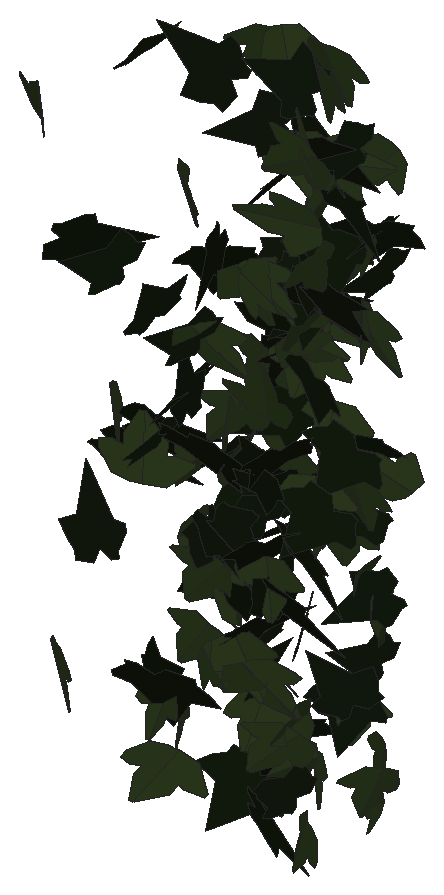
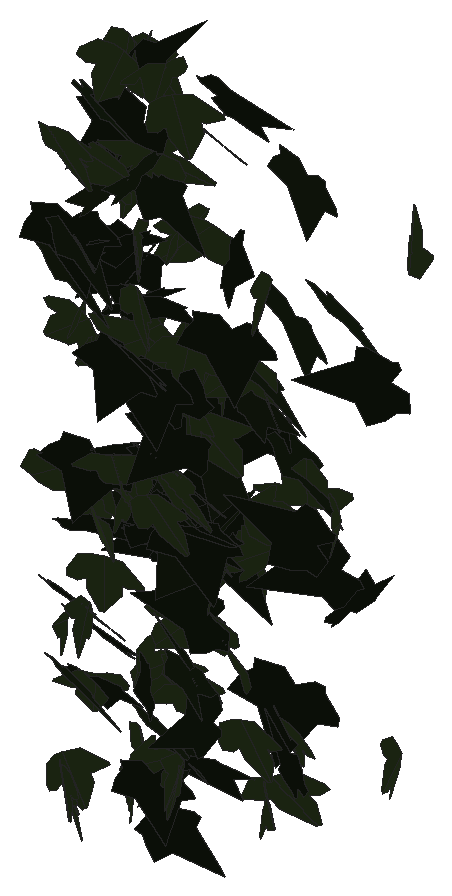
# SketchUp Ruby script. Lengths in inches.
U = 1.inch
M = Sketchup.active_model
def pt(a) = Geom::Point3d.new(a.map { |v| v * U })
def face(e, loops, mat)
  f = e.add_face(loops[0].map { |a| pt(a) })
  loops[1..].each { |l| e.add_face(l.map { |a| pt(a) }).erase! }
  f.material = f.back_material = mat if mat
  f
end
# faces: each face lists its corners as indices into pts; further lists are holes
def faces(e, pts, list, mat = nil) = list.each { |f| face(e, (f[0].is_a?(Array) ? f : [f]).map { |l| l.map { |i| pts[i] } }, mat) }
# xy, xz, yz: faces in a plane at the given z, y or x. An outline is a flat list of corners, or four numbers for a rectangle; further outlines are holes
def ring(l) = l.size == 4 ? [[l[0], l[1]], [l[2], l[1]], [l[2], l[3]], [l[0], l[3]]] : l.each_slice(2).to_a
def flat(e, list, mat, &to3) = list.each { |f| face(e, (f[0].is_a?(Array) ? f : [f]).map { |l| ring(l).map { |u, v| to3.(u, v) } }, mat) }
def xy(e, z, list, mat = nil) = flat(e, list, mat) { |x, y| [x, y, z] }
def xz(e, y, list, mat = nil) = flat(e, list, mat) { |x, z| [x, y, z] }
def yz(e, x, list, mat = nil) = flat(e, list, mat) { |y, z| [x, y, z] }
def lines(e, pts, list) = list.each { |a, b| e.add_line(pt(pts[a]), pt(pts[b])) }
# prism: a flat outline (further loops are holes) pulled along v
def prism(e, loops, v, mat = nil)
  f = face(e, loops, mat); d = Geom::Vector3d.new(v.map { |x| x * U })
  f.pushpull(f.normal.samedirection?(d) ? d.length : -d.length)
end
def box(e, o, s, mat = nil) = prism(e, [[o, [o[0] + s[0], o[1], o[2]], [o[0] + s[0], o[1] + s[1], o[2]], [o[0], o[1] + s[1], o[2]]]], [0, 0, s[2]], mat)
def at(x, y, z, deg = 0) = Geom::Transformation.translation(pt([x, y, z])) * Geom::Transformation.rotation(ORIGIN, Z_AXIS, deg.degrees)
def axes(o, x, y, z) = Geom::Transformation.new([*x, 0, *y, 0, *z, 0, *pt(o).to_a, 1])
def part(name) = M.definitions.add(name)
# library, detail: a bought-in or finely detailed component or shape, given as its bounding box
def library(name, o, s) = part(name).tap { |d| box(d.entities, o, s) }
def detail(e, o, s) = box(e.add_group.entities, o, s)
def put(e, d, t, mat = nil) = e.add_instance(d, t).tap { |i| i.material = mat if mat }
def group(e, t, mat = nil) = e.add_group.tap { |g| g.transformation = t; g.material = mat if mat }.entities
root = M.entities
M.materials.add("1026 AP 7946 SUNNY SIDE UP").color = [254, 231, 186]
M.materials.add("efeu1").color = [18, 25, 13]
M.materials.add("efeu2").color = [43, 57, 29]
c1 = part("ivyleaf_9")
p = [[1.54,2.16,1.25],[1.36,2.04,1.19],[-0.21,0.99,0.68],[-0.71,1.11,0.82],[-0.85,0.86,0.67],[-0.8,0.17,0.21],
  [-0.9,-0.01,0.1],[-0.67,-0.16,-0.02],[-0.08,-0.08,-0.05],[-0.03,-0.6,-0.4],[0.65,-0.88,-0.66],[0.83,-0.6,-0.49],
  [1.29,-0.42,-0.43],[1.8125,-0.07,-0.26],[1.21,0.44,0.15]]
faces(c1.entities,p,[[0,1,2,3,4,5,6,7,8,9,10,11,12,13,14]],"efeu1")
c2 = part("ivyleaf_10")
p = [[0,0.5,-0.03],[-0.0625,2.02,-0.43],[-0.19,2.01,-0.46],[-0.54,1.05,-0.29],[-0.52,0.625,-0.18],[-0.83,0.76,-0.28],
  [-1.16,0.64,-0.33],[-1.15,0.33,-0.24],[-0.77,-0.39,0.02],[-0.3,-0.51,0.16],[0.04,-0.48,0.23],[-0.02,2.01,-0.4375],
  [-0.06,2.01,-0.43],[0.04,-0.49,0.23],[0.67,-0.49,0.14],[1.38,0.36,-0.2],[1.375,0.51,-0.24],[0.81,0.65,-0.19],
  [0.62,0.59,-0.15],[0.6,1.09,-0.28],[0.5,1.23,-0.31]]
faces(c2.entities,p,[[0,1,2,3,4,5,6,7,8,9,10],[11,12,0,13,14,15,16,17,18,19,20]],"efeu2")
put(root,c1,axes([97.57,211.43,285.4],[-0.02383,0.29282,-0.12965],[0.02278,-0.12438,-0.3155],[-0.53994,-0.01817,-0.00759]),"1026 AP 7946 SUNNY SIDE UP")
put(root,c1,axes([96.1,211.34,285.11],[0.5804,0.06021,-0.09484],[-0.15726,0.01233,-0.37035],[-0.09346,0.35318,0.03417]),"1026 AP 7946 SUNNY SIDE UP")
put(root,c1,axes([95.49,211.43,284.89],[-0.25342,0.29453,-0.03914],[0.00462,-0.04385,-0.35364],[-0.50464,-0.14831,0.01642]),"1026 AP 7946 SUNNY SIDE UP")
put(root,c1,axes([95.49,211.38,281.24],[0.47591,0.14978,-0.1513],[-0.20633,-0.07643,-0.34121],[-0.28502,0.30543,-0.00564]),"1026 AP 7946 SUNNY SIDE UP")
put(root,c2,axes([97.57,211.62,280.87],[-0.33154,-0.14288,0.2048],[-0.19603,-0.16247,-0.25593],[0.35766,-0.2215,0.04957]),"1026 AP 7946 SUNNY SIDE UP")
put(root,c1,axes([94.84,211.4,287.32],[-0.2851,0.26757,0.10404],[-0.1298,0.06211,-0.33577],[-0.46342,-0.18201,0.03004]),"1026 AP 7946 SUNNY SIDE UP")
put(root,c2,axes([96.43,211.53,283.13],[-0.47339,-0.03717,0.17911],[-0.26834,-0.07,-0.29885],[0.11445,-0.31784,0.04016]),"1026 AP 7946 SUNNY SIDE UP")
put(root,c2,axes([95.54,211.59,279.86],[0.45236,0.12368,-0.16682],[-0.23003,-0.08151,-0.31525],[-0.25018,0.29859,-0.01177]),"1026 AP 7946 SUNNY SIDE UP")
put(root,c2,axes([97.2,211.57,283.4],[0.50584,-0.01989,0.0995],[0.15538,-0.0254,-0.31947],[0.04502,0.31118,-0.01533]),"1026 AP 7946 SUNNY SIDE UP")
put(root,c2,axes([93.66,211.55,280.87],[-0.26233,0.27662,-0.11767],[0.04788,-0.11372,-0.33938],[-0.50531,-0.15438,0.02893]),"1026 AP 7946 SUNNY SIDE UP")
put(root,c2,axes([97.07,211.49,281.8],[-0.42943,-0.09787,-0.19649],[0.31475,0.02044,-0.28698],[0.15577,-0.31112,0.03817]),"1026 AP 7946 SUNNY SIDE UP")
put(root,c1,axes([97.17,211.46,279.73],[0.39889,-0.1767,-0.18172],[-0.20291,0.11898,-0.31235],[0.35999,0.26286,0.02531]),"1026 AP 7946 SUNNY SIDE UP")
put(root,c2,axes([97.97,211.51,290.03],[-0.35651,0.0191,0.27204],[-0.43213,-0.01927,-0.22418],[0.00462,-0.32891,0.02431]),"1026 AP 7946 SUNNY SIDE UP")
put(root,c2,axes([97.98,211.51,279.65],[-0.29823,0.25671,0.06959],[-0.22701,-0.02267,-0.3072],[-0.38643,-0.1848,0.12676]),"1026 AP 7946 SUNNY SIDE UP")
put(root,c1,axes([97.26,211.47,284.99],[0.0507,-0.00402,-0.33283],[-0.52764,-0.00502,-0.03198],[-0.00784,0.31222,-0.00044]),"1026 AP 7946 SUNNY SIDE UP")
put(root,c2,axes([96.73,211.35,285.44],[0.14773,-0.03586,0.33108],[-0.3063,0.25646,0.08964],[-0.43165,-0.19425,0.0497]),"1026 AP 7946 SUNNY SIDE UP")
put(root,c2,axes([95.38,211.64,280.81],[0.39832,-0.18079,0.05152],[0.04098,-0.05103,-0.31979],[0.29252,0.25332,-0.02535]),"1026 AP 7946 SUNNY SIDE UP")
put(root,c1,axes([97.26,211.49,283.84],[0.06219,0.2906,-0.11568],[-0.01617,-0.11151,-0.31509],[-0.52833,0.03762,-0.00397]),"1026 AP 7946 SUNNY SIDE UP")
put(root,c1,axes([94.42,211.48,282.85],[-0.25922,-0.19832,0.25839],[0.21486,0.20946,0.27006],[-0.48852,0.19736,-0.01833]),"1026 AP 7946 SUNNY SIDE UP")
put(root,c2,axes([95.15,211.5,284.28],[0.50666,0.18275,-0.03413],[0.01917,0.04687,0.37357],[0.31506,-0.29675,0.03217]),"1026 AP 7946 SUNNY SIDE UP")
put(root,c2,axes([96.66,211.66,281.97],[0.4227,0.0199,0.19991],[0.31831,-0.03134,-0.26492],[0.00505,0.30951,-0.0353]),"1026 AP 7946 SUNNY SIDE UP")
put(root,c1,axes([96.23,211.62,283.77],[0.25995,-0.26719,-0.10353],[-0.09025,0.08086,-0.32315],[0.43885,0.1749,-0.00513]),"1026 AP 7946 SUNNY SIDE UP")
put(root,c1,axes([96.54,211.5625,283.08],[0.15257,0.04294,-0.32039],[-0.48542,-0.09109,-0.107],[-0.16953,0.29946,0.01804]),"1026 AP 7946 SUNNY SIDE UP")
put(root,c1,axes([97.26,211.6,283.05],[0.4902,-0.1036,0.07593],[0.10051,-0.0483,-0.32804],[0.18942,0.29373,-0.02244]),"1026 AP 7946 SUNNY SIDE UP")
put(root,c1,axes([95.48,211.35,286.82],[-0.00603,0.27813,0.24511],[-0.06193,0.22388,-0.29334],[-0.60447,-0.02571,0.02761]),"1026 AP 7946 SUNNY SIDE UP")
put(root,c2,axes([96.06,211.8125,281.56],[-0.15125,-0.02784,-0.30461],[0.23001,-0.26615,-0.02128],[-0.42663,-0.13362,0.09652]),"1026 AP 7946 SUNNY SIDE UP")
put(root,c1,axes([95.98,211.42,285.54],[0.052,0.05241,0.35166],[-0.03712,0.32879,-0.0495],[-0.56229,-0.01686,0.03579]),"1026 AP 7946 SUNNY SIDE UP")
put(root,c2,axes([97.05,211.47,287.83],[-0.04722,0.27411,0.21362],[-0.02731,0.20511,-0.28284],[-0.53828,-0.03445,-0.00439]),"1026 AP 7946 SUNNY SIDE UP")
put(root,c1,axes([97.68,211.59,280.07],[-0.2149,0.23966,0.12776],[-0.15333,0.08242,-0.28615],[-0.42536,-0.15079,0.0386]),"1026 AP 7946 SUNNY SIDE UP")
put(root,c2,axes([97.97,211.64,288.4],[-0.10616,-0.29211,-0.15921],[0.07828,0.13814,-0.3175],[0.54796,-0.07633,0.01451]),"1026 AP 7946 SUNNY SIDE UP")
put(root,c2,axes([97.57,211.95,281.0625],[0.00454,0.06454,-0.33927],[-0.1375,-0.30754,-0.0719],[-0.53294,0.0799,0.01566]),"1026 AP 7946 SUNNY SIDE UP")
put(root,c2,axes([96.82,211.67,287.77],[-0.34879,-0.15368,-0.21458],[0.34076,0.03773,-0.26734],[0.22054,-0.30133,0.07371]),"1026 AP 7946 SUNNY SIDE UP")
put(root,c1,axes([97.29,211.59,282.88],[-0.08507,-0.13222,0.29605],[0.31333,0.21283,0.14682],[-0.41871,0.18612,0.04972]),"1026 AP 7946 SUNNY SIDE UP")
put(root,c1,axes([96.31,211.63,283.76],[0.04627,-0.16902,-0.31337],[-0.07722,0.28692,-0.17928],[0.56529,0.05303,0.00116]),"1026 AP 7946 SUNNY SIDE UP")
put(root,c2,axes([97.89,211.6875,289.875],[-0.2263,0.28694,-0.0747],[-0.0419,0.06958,0.33962],[0.50108,0.13541,-0.00534]),"1026 AP 7946 SUNNY SIDE UP")
put(root,c1,axes([96.78,211.92,279.91],[-0.48372,-0.13016,-0.01357],[0.03751,-0.02208,-0.33422],[0.21854,-0.28431,0.02735]),"1026 AP 7946 SUNNY SIDE UP")
put(root,c1,axes([95.85,211.94,285.81],[-0.33289,0.09448,-0.24321],[0.22664,-0.20488,-0.2163],[-0.35312,-0.22056,0.09045]),"1026 AP 7946 SUNNY SIDE UP")
put(root,c2,axes([97.63,211.82,288.76],[0.10723,-0.01823,-0.3408],[-0.53599,0.03989,-0.06902],[0.0725,0.32185,-0.00618]),"1026 AP 7946 SUNNY SIDE UP")
put(root,c2,axes([96.99,211.83,285.69],[-0.52504,0.06341,0.00538],[0.01562,0.02404,0.33725],[0.10673,0.30838,-0.02289]),"1026 AP 7946 SUNNY SIDE UP")
put(root,c1,axes([97.44,212,283.69],[0.2172,-0.28419,0.11491],[0.07301,-0.10241,-0.33508],[0.51277,0.13496,-0.00097]),"1026 AP 7946 SUNNY SIDE UP")
put(root,c2,axes([96.53,211.71,282.48],[-0.05518,0.27726,-0.1695],[-0.02231,0.16148,0.30107],[0.5446,0.03471,-0.00484]),"1026 AP 7946 SUNNY SIDE UP")
put(root,c1,axes([95.99,212.07,287.82],[-0.07845,0.02451,-0.34969],[0.38901,-0.23373,-0.05669],[-0.39806,-0.23325,0.01351]),"1026 AP 7946 SUNNY SIDE UP")
put(root,c2,axes([93.01,211.9375,288.8],[-0.35262,0.22801,0.13645],[0.17647,-0.07311,0.32805],[0.40413,0.23087,-0.02419]),"1026 AP 7946 SUNNY SIDE UP")
put(root,c2,axes([96.82,211.95,281],[0.34252,0.2017,-0.10164],[-0.09768,-0.08025,-0.30612],[-0.36759,0.20927,-0.01336]),"1026 AP 7946 SUNNY SIDE UP")
put(root,c1,axes([97.875,212.13,284.28],[-0.37347,-0.17954,0.07847],[-0.0591,-0.07602,-0.30266],[0.32539,-0.21987,0.03509]),"1026 AP 7946 SUNNY SIDE UP")
put(root,c2,axes([95.44,212.2,284.21],[0.01066,-0.06601,0.32114],[-0.00028,-0.30089,-0.07488],[0.52282,0.00119,-0.00659]),"1026 AP 7946 SUNNY SIDE UP")
put(root,c1,axes([96.58,211.75,282.09],[0.04885,0.28023,-0.15848],[0.01325,0.15164,0.30361],[0.54075,-0.02903,0.00688]),"1026 AP 7946 SUNNY SIDE UP")
put(root,c2,axes([96.4,211.78,284.6],[0.13641,-0.12802,0.30171],[-0.12439,0.27677,0.1599],[-0.51317,-0.10111,0.04144]),"1026 AP 7946 SUNNY SIDE UP")
put(root,c2,axes([95.78,211.77,283.34],[0.01723,0.0031,0.33061],[-0.02523,0.30858,0.00151],[-0.52357,-0.01477,0.01081]),"1026 AP 7946 SUNNY SIDE UP")
put(root,c1,axes([95.76,211.92,286.29],[-0.24116,0.2755,0.0798],[-0.10378,0.04789,-0.32946],[-0.47165,-0.1514,0.03169]),"1026 AP 7946 SUNNY SIDE UP")
put(root,c1,axes([96.57,212.01,281.25],[-0.07591,0.25934,0.1731],[0.06055,-0.15443,0.27947],[0.51221,0.05669,-0.00738]),"1026 AP 7946 SUNNY SIDE UP")
put(root,c2,axes([95.73,212.06,286.28],[-0.38873,-0.10758,-0.20078],[0.3186,0.03262,-0.26692],[0.17802,-0.2933,0.03926]),"1026 AP 7946 SUNNY SIDE UP")
put(root,c1,axes([97.43,212.35,286.08],[-0.03618,-0.21963,0.21452],[0.05102,-0.2043,-0.23583],[0.5054,0.00491,0.03916]),"1026 AP 7946 SUNNY SIDE UP")
put(root,c1,axes([97.01,212.14,289.9375],[-0.4241,0.18621,0.06294],[-0.12357,-0.00439,-0.32995],[-0.30628,-0.25608,0.04597]),"1026 AP 7946 SUNNY SIDE UP")
put(root,c2,axes([94.05,212.29,284.65],[-0.13981,0.19014,-0.24438],[0.08364,-0.22744,-0.22264],[-0.50061,-0.0911,0.03105]),"1026 AP 7946 SUNNY SIDE UP")
put(root,c1,axes([94.71,212.3125,280.49],[-0.01063,0.08493,0.31029],[0.10395,-0.28239,0.08641],[0.5002,0.06049,-0.01137]),"1026 AP 7946 SUNNY SIDE UP")
put(root,c2,axes([96.27,212.31,285.26],[-0.31533,-0.18393,0.189],[-0.17591,-0.14948,-0.27966],[0.36996,-0.22785,0.02812]),"1026 AP 7946 SUNNY SIDE UP")
put(root,c1,axes([97.29,212.4,290.43],[-0.09876,0.05714,0.34641],[-0.4193,-0.22323,-0.00847],[0.36594,-0.24036,0.08378]),"1026 AP 7946 SUNNY SIDE UP")
put(root,c2,axes([97.73,212.27,283.98],[0.24004,-0.25414,0.01732],[-0.00334,-0.02338,-0.31137],[0.43267,0.14081,-0.01201]),"1026 AP 7946 SUNNY SIDE UP")
put(root,c1,axes([98.26,212.11,281.49],[-0.01801,0.18007,0.24597],[-0.30146,0.1759,-0.15553],[-0.38934,-0.14452,0.10905]),"1026 AP 7946 SUNNY SIDE UP")
put(root,c1,axes([96.07,212.18,290.3125],[-0.41473,-0.01039,-0.24549],[-0.38818,-0.01578,0.26153],[-0.03118,0.3346,0.00939]),"1026 AP 7946 SUNNY SIDE UP")
put(root,c1,axes([96.15,212.06,284.625],[0.10327,0.25646,0.17757],[0.00375,0.16537,-0.27795],[-0.51539,0.05259,0.03356]),"1026 AP 7946 SUNNY SIDE UP")
put(root,c1,axes([96.71,212.16,283.74],[-0.16694,0.23493,0.1805],[-0.1661,0.13714,-0.26868],[-0.45871,-0.13516,0.0316]),"1026 AP 7946 SUNNY SIDE UP")
put(root,c1,axes([97.48,212.22,287.49],[0.50476,0.07106,0.00475],[0.01835,-0.03021,-0.32593],[-0.11937,0.29583,-0.03001]),"1026 AP 7946 SUNNY SIDE UP")
put(root,c2,axes([97.11,212.55,280.01],[0.01445,-0.00846,0.31127],[0.02034,-0.29073,-0.01348],[0.49354,0.01223,-0.00856]),"1026 AP 7946 SUNNY SIDE UP")
put(root,c1,axes([93.34,212.1,286.92],[0.13183,0.16652,-0.28881],[0.05548,0.27426,0.19361],[0.53845,-0.06903,0.05076]),"1026 AP 7946 SUNNY SIDE UP")
put(root,c2,axes([97.375,212.39,284.35],[0.40987,0.17385,-0.03234],[-0.01824,-0.04043,-0.31784],[-0.29967,0.24024,-0.02488]),"1026 AP 7946 SUNNY SIDE UP")
put(root,c2,axes([97.43,212.6,288.875],[0.02943,-0.11847,0.32394],[0.15839,-0.29004,-0.1307],[0.53093,0.09309,0.02104]),"1026 AP 7946 SUNNY SIDE UP")
put(root,c2,axes([97.22,212.3,286.58],[-0.02942,-0.2752,0.18655],[0.01388,0.17767,0.29767],[-0.55604,0.019,-0.00244]),"1026 AP 7946 SUNNY SIDE UP")
put(root,c1,axes([94.03,212.29,283.9375],[0.46684,0.06222,0.1539],[0.25108,-0.01254,-0.29898],[-0.08362,0.30969,-0.03853]),"1026 AP 7946 SUNNY SIDE UP")
put(root,c2,axes([95.05,212.52,280.16],[-0.16076,0.24891,-0.15242],[-0.05149,-0.16724,-0.26499],[-0.45353,-0.06924,0.08411]),"1026 AP 7946 SUNNY SIDE UP")
put(root,c1,axes([94.33,212.41,284.28],[0.36597,0.08842,-0.21314],[0.28836,0.10967,0.24917],[0.23434,-0.27303,0.02624]),"1026 AP 7946 SUNNY SIDE UP")
put(root,c1,axes([98.07,212.46,289.79],[-0.37329,0.22377,0.00794],[-0.04141,-0.01769,-0.33461],[-0.37768,-0.21923,0.02884]),"1026 AP 7946 SUNNY SIDE UP")
put(root,c1,axes([97.17,212.44,287.59],[0.26358,-0.18705,-0.21017],[-0.19927,0.15444,-0.25801],[0.41162,0.19455,0.00968]),"1026 AP 7946 SUNNY SIDE UP")
put(root,c1,axes([97.3,212.36,289.55],[0.47572,0.14542,0.08187],[0.13583,0.00079,-0.34384],[-0.22164,0.3126,-0.03499]),"1026 AP 7946 SUNNY SIDE UP")
put(root,c2,axes([97.49,212.46,290.71],[-0.4009,0.23123,0.05553],[-0.09673,0.01008,-0.35285],[-0.36011,-0.26013,0.03296]),"1026 AP 7946 SUNNY SIDE UP")
put(root,c1,axes([96.42,212.39,281.59],[-0.06004,0.27612,0.09265],[-0.05097,0.07958,-0.29623],[-0.48676,-0.04239,0.01959]),"1026 AP 7946 SUNNY SIDE UP")
put(root,c2,axes([97.08,212.42,286.53],[-0.17642,-0.13434,-0.28128],[0.32233,0.18036,-0.17782],[0.37998,-0.21537,0.02025]),"1026 AP 7946 SUNNY SIDE UP")
put(root,c1,axes([96.51,212.34,283.34],[0.20344,0.22771,0.16373],[0.06333,0.14858,-0.27137],[-0.45849,0.12156,0.03517]),"1026 AP 7946 SUNNY SIDE UP")
put(root,c1,axes([97.79,212.74,281.18],[-0.37856,-0.10843,-0.13595],[0.22872,0.0044,-0.26017],[0.16433,-0.25589,0.04892]),"1026 AP 7946 SUNNY SIDE UP")
put(root,c2,axes([97.09,212.68,286.21],[0.47376,0.09991,-0.06155],[-0.07583,-0.04876,-0.31638],[-0.1816,0.28102,-0.02847]),"1026 AP 7946 SUNNY SIDE UP")
put(root,c2,axes([97.79,212.66,281.13],[0.35927,0.18007,-0.00185],[0.01806,-0.01878,-0.29689],[-0.30522,0.21084,-0.01975]),"1026 AP 7946 SUNNY SIDE UP")
put(root,c1,axes([96.81,212.66,288.99],[-0.20499,0.25942,-0.1644],[0.07898,-0.15108,-0.30779],[-0.50861,-0.12802,0.01847]),"1026 AP 7946 SUNNY SIDE UP")
put(root,c1,axes([96.29,212.81,283.95],[-0.48785,-0.09225,0.02536],[-0.02398,-0.03653,-0.33218],[0.14842,-0.30913,0.0297]),"1026 AP 7946 SUNNY SIDE UP")
put(root,c2,axes([96.89,212.68,289.34],[0.49155,0.11193,0.10658],[0.17478,0.00431,-0.33058],[-0.18245,0.3057,-0.02953]),"1026 AP 7946 SUNNY SIDE UP")
put(root,c1,axes([96.99,212.89,287.22],[-0.1697,-0.31927,0.04957],[0.00837,-0.05439,-0.34676],[0.50806,-0.10574,0.02227]),"1026 AP 7946 SUNNY SIDE UP")
put(root,c1,axes([96.79,212.79,284.1],[-0.04192,0.16146,-0.2596],[0.01485,-0.24494,-0.17747],[-0.49729,-0.02093,0.01658]),"1026 AP 7946 SUNNY SIDE UP")
put(root,c2,axes([95.23,212.74,281.25],[-0.43312,0.04552,0.14257],[-0.22849,-0.07402,-0.27383],[-0.00937,-0.29912,0.08756]),"1026 AP 7946 SUNNY SIDE UP")
put(root,c1,axes([96.93,212.73,286.12],[0.04891,0.24089,-0.18938],[-0.05404,-0.1774,-0.26205],[-0.50764,0.04209,0.00965]),"1026 AP 7946 SUNNY SIDE UP")
put(root,c1,axes([97.63,212.97,284.76],[-0.29949,-0.21565,0.12139],[-0.04032,-0.12746,-0.29364],[0.41387,-0.16847,0.05924]),"1026 AP 7946 SUNNY SIDE UP")
put(root,c1,axes([97.29,212.9,288.02],[-0.18418,-0.29627,-0.03491],[0.03155,0.0238,-0.3373],[0.50431,-0.10969,0.00835]),"1026 AP 7946 SUNNY SIDE UP")
put(root,c2,axes([97.07,212.86,279.81],[-0.20228,0.18095,-0.17772],[0.04076,-0.17754,-0.22496],[-0.41758,-0.10498,0.06413]),"1026 AP 7946 SUNNY SIDE UP")
put(root,c1,axes([95.5,212.68,287.18],[0.24985,0.24699,-0.11971],[-0.06278,-0.11143,-0.30834],[-0.45823,0.14993,-0.02303]),"1026 AP 7946 SUNNY SIDE UP")
put(root,c2,axes([96.22,212.77,285.82],[-0.46807,0.12431,0.0684],[-0.14043,-0.04838,-0.32289],[-0.17075,-0.30098,0.07805]),"1026 AP 7946 SUNNY SIDE UP")
put(root,c2,axes([96.58,212.78,290.82],[0.19834,0.30098,-0.01557],[0.00891,-0.02183,-0.34568],[-0.51181,0.11626,-0.01205]),"1026 AP 7946 SUNNY SIDE UP")
put(root,c1,axes([97.35,212.91,288.84],[0.23336,-0.31255,0.02206],[0.02077,-0.0194,-0.35654],[0.49237,0.14896,0.00459]),"1026 AP 7946 SUNNY SIDE UP")
put(root,c2,axes([94.89,212.74,288.0625],[-0.2639,0.27197,0.04417],[-0.05304,0.02553,-0.33466],[-0.46306,-0.15792,0.01316]),"1026 AP 7946 SUNNY SIDE UP")
put(root,c1,axes([96.03,212.78,284.01],[0.26631,0.1717,-0.1924],[-0.20319,-0.13708,-0.25088],[-0.37293,0.1973,-0.0007]),"1026 AP 7946 SUNNY SIDE UP")
put(root,c1,axes([94.29,212.61,289.92],[0.05079,0.28856,0.16141],[-0.01406,0.14827,-0.30769],[-0.54956,0.02287,0.02279]),"1026 AP 7946 SUNNY SIDE UP")
put(root,c1,axes([96.42,212.94,279.57],[-0.12224,0.16281,-0.2218],[-0.03206,-0.21947,-0.17888],[-0.44898,-0.02866,0.07316]),"1026 AP 7946 SUNNY SIDE UP")
put(root,c2,axes([98.03,212.95,279.89],[-0.19998,-0.26888,0.08373],[-0.01215,-0.0875,-0.30544],[0.44221,-0.124,0.02948]),"1026 AP 7946 SUNNY SIDE UP")
put(root,c2,axes([97.78,212.99,286.93],[-0.07333,0.24621,-0.17913],[-0.0027,-0.17248,-0.26858],[-0.5084,-0.0346,0.02726]),"1026 AP 7946 SUNNY SIDE UP")
put(root,c2,axes([96.81,213.01,288.24],[0.17555,-0.30142,0.10647],[0.1722,-0.06837,-0.32238],[0.47145,0.13721,0.07811]),"1026 AP 7946 SUNNY SIDE UP")
put(root,c1,axes([96.6875,213.02,287.4375],[-0.26198,-0.21704,-0.20165],[0.29363,0.09251,-0.2706],[0.35184,-0.23882,0.07568]),"1026 AP 7946 SUNNY SIDE UP")
put(root,c2,axes([97.27,212.9,290.76],[-0.508,0.10685,-0.05701],[0.07329,-0.04114,-0.3398],[-0.19008,-0.30141,0.02136]),"1026 AP 7946 SUNNY SIDE UP")
put(root,c2,axes([97.32,212.95,289.12],[0.16265,-0.08904,-0.31302],[0.48629,-0.07722,0.1251],[-0.17539,-0.29669,0.05659]),"1026 AP 7946 SUNNY SIDE UP")
put(root,c1,axes([95.66,212.93,281.33],[0.4107,-0.17643,0.0065],[0.00486,-0.00848,-0.32472],[0.27761,0.26116,-0.00393]),"1026 AP 7946 SUNNY SIDE UP")
put(root,c1,axes([96.64,212.97,285.05],[-0.47282,0.13486,0.02969],[-0.06124,-0.01864,-0.33793],[-0.20775,-0.30143,0.03206]),"1026 AP 7946 SUNNY SIDE UP")
put(root,c2,axes([96.05,212.93,286.8],[-0.46545,-0.11384,-0.03461],[0.06501,-0.01211,-0.31681],[0.18936,-0.27565,0.0237]),"1026 AP 7946 SUNNY SIDE UP")
put(root,c2,axes([97.67,212.96,284.26],[-0.47681,0.09975,-0.02889],[0.03297,-0.02962,-0.31871],[-0.1729,-0.28075,0.0189]),"1026 AP 7946 SUNNY SIDE UP")
put(root,c2,axes([96.5625,213,284.3],[-0.38036,0.04908,0.18429],[-0.30282,-0.06131,-0.23158],[-0.00037,-0.27542,0.08024]),"1026 AP 7946 SUNNY SIDE UP")
put(root,c1,axes([96.61,212.91,280.18],[0.14158,0.24727,-0.09657],[-0.03902,-0.09081,-0.28055],[-0.44702,0.08624,-0.0061]),"1026 AP 7946 SUNNY SIDE UP")
put(root,c1,axes([96.03,213.1,286.02],[-0.00817,-0.04688,0.33656],[0.39002,-0.2165,-0.02919],[0.34299,0.24507,0.04121]),"1026 AP 7946 SUNNY SIDE UP")
put(root,c1,axes([97.65,213.18,283.8],[-0.43059,-0.10178,0.09731],[-0.11387,-0.07721,-0.28983],[0.20346,-0.25862,0.04374]),"1026 AP 7946 SUNNY SIDE UP")
put(root,c2,axes([97.78,213.08,286.72],[-0.35286,0.10505,-0.21079],[0.25324,-0.13718,-0.24717],[-0.28452,-0.25239,0.04143]),"1026 AP 7946 SUNNY SIDE UP")
put(root,c2,axes([97.76,213.0625,287.91],[0.25566,-0.26832,-0.03338],[-0.05308,0.01413,-0.3285],[0.45481,0.15248,-0.01957]),"1026 AP 7946 SUNNY SIDE UP")
put(root,c1,axes([98.05,213.14,282.62],[-0.46447,0.07602,-0.01223],[0.00009,-0.04564,-0.301],[-0.13075,-0.27006,0.04325]),"1026 AP 7946 SUNNY SIDE UP")
put(root,c2,axes([96.92,213.21,284.4],[-0.08321,0.20804,-0.20935],[-0.06007,-0.20396,-0.22261],[-0.48413,-0.01045,0.0636]),"1026 AP 7946 SUNNY SIDE UP")
put(root,c2,axes([96.07,213.125,290.55],[-0.32761,-0.24404,0.05417],[-0.02994,-0.05448,-0.33318],[0.42314,-0.1928,0.01836]),"1026 AP 7946 SUNNY SIDE UP")
put(root,c2,axes([98,212.98,279.47],[0.11156,-0.18104,-0.21332],[-0.14241,0.17857,-0.20326],[0.43114,0.10583,-0.01194]),"1026 AP 7946 SUNNY SIDE UP")
put(root,c1,axes([96.62,213.21,289.37],[0.20332,-0.28385,0.03126],[0.00626,-0.03413,-0.33014],[0.48504,0.11943,-0.00884]),"1026 AP 7946 SUNNY SIDE UP")
put(root,c2,axes([96.18,213.02,280.39],[-0.28052,0.20331,0.09016],[-0.10107,0.05664,-0.2795],[-0.35787,-0.17536,0.00827]),"1026 AP 7946 SUNNY SIDE UP")
put(root,c2,axes([96.93,212.95,286.67],[0.27421,0.09288,0.28246],[0.27714,0.21911,-0.19104],[-0.3601,0.23935,0.06806]),"1026 AP 7946 SUNNY SIDE UP")
put(root,c2,axes([98.07,213.11,289.4],[0.40961,-0.15369,-0.13512],[-0.18838,0.05681,-0.30526],[0.27755,0.26537,-0.00779]),"1026 AP 7946 SUNNY SIDE UP")
put(root,c2,axes([96.22,212.92,280.42],[-0.00152,0.14163,0.25946],[-0.1851,0.22122,-0.13681],[-0.43615,-0.09438,0.05716]),"1026 AP 7946 SUNNY SIDE UP")
put(root,c1,axes([96.69,212.92,281.47],[0.024,0.02683,0.29436],[0.10895,0.2671,-0.02775],[-0.45552,0.0653,0.00888]),"1026 AP 7946 SUNNY SIDE UP")
put(root,c1,axes([98.12,213.1,287.64],[-0.28677,0.25439,-0.01735],[-0.00504,-0.02537,-0.32681],[-0.43308,-0.16815,0.01529]),"1026 AP 7946 SUNNY SIDE UP")
put(root,c2,axes([98.18,213.22,284.35],[0.21139,0.15086,0.23323],[-0.27016,-0.14718,0.20633],[0.35624,-0.20113,0.01807]),"1026 AP 7946 SUNNY SIDE UP")
put(root,c1,axes([97.84,213.11,288.23],[0.25978,0.21478,-0.16974],[-0.13923,-0.13947,-0.28398],[-0.43424,0.17321,-0.01049]),"1026 AP 7946 SUNNY SIDE UP")
put(root,c1,axes([97.82,213.125,288.07],[-0.17103,0.29145,-0.01808],[-0.00386,-0.02266,-0.33029],[-0.49598,-0.10033,0.0088]),"1026 AP 7946 SUNNY SIDE UP")
put(root,c1,axes([96.76,213.32,286.72],[-0.47486,0.06611,-0.08183],[0.11894,-0.03873,-0.30746],[-0.12516,-0.28762,0.01829]),"1026 AP 7946 SUNNY SIDE UP")
put(root,c1,axes([97.4375,213.13,284.8],[0.38945,0.16524,-0.07983],[-0.11608,-0.03625,-0.303],[-0.28665,0.23917,0.01424]),"1026 AP 7946 SUNNY SIDE UP")
put(root,c2,axes([97.25,213.3,284.09],[0.12628,-0.27728,0.00093],[-0.01566,-0.00711,-0.30724],[0.4705,0.07418,-0.01047]),"1026 AP 7946 SUNNY SIDE UP")
put(root,c1,axes([96.52,213.2,286.38],[0.32047,0.15462,-0.18458],[-0.20694,-0.12582,-0.26241],[-0.33725,0.22413,-0.01438]),"1026 AP 7946 SUNNY SIDE UP")
put(root,c2,axes([96.97,213.3,284.98],[0.41014,0.15215,-0.04705],[-0.03939,-0.0489,-0.30481],[-0.2669,0.24102,-0.02731]),"1026 AP 7946 SUNNY SIDE UP")
put(root,c1,axes([95.91,213.18,285.7],[0.50978,0.05171,-0.01757],[-0.01608,-0.0451,-0.33558],[-0.08425,0.32152,-0.04228]),"1026 AP 7946 SUNNY SIDE UP")
put(root,c2,axes([97.19,213.28,283.3],[-0.46667,-0.05943,0.02112],[-0.02225,-0.03579,-0.29964],[0.10438,-0.27334,0.03058]),"1026 AP 7946 SUNNY SIDE UP")
put(root,c2,axes([97.96,213.06,282.12],[-0.00693,0.10029,-0.28812],[0.00876,0.27044,0.11106],[0.48955,-0.00342,-0.00606]),"1026 AP 7946 SUNNY SIDE UP")
put(root,c2,axes([96.09,213.2,284.91],[0.17997,-0.12783,-0.28672],[-0.34805,0.1697,-0.17354],[0.33132,0.2477,-0.02656]),"1026 AP 7946 SUNNY SIDE UP")
put(root,c1,axes([97.84,213.22,281.47],[-0.23979,0.21432,0.11637],[-0.13775,0.07272,-0.27241],[-0.38171,-0.16087,0.0252]),"1026 AP 7946 SUNNY SIDE UP")
put(root,c2,axes([96.63,213.29,287.55],[-0.34839,0.19922,0.10378],[-0.22022,-0.00494,-0.29102],[-0.30253,-0.22582,0.09232]),"1026 AP 7946 SUNNY SIDE UP")
put(root,c2,axes([97.74,213.38,280.01],[0.25565,-0.20961,-0.08053],[0.00249,0.08856,-0.26965],[0.37648,0.14175,0.05647]),"1026 AP 7946 SUNNY SIDE UP")
put(root,c1,axes([96.78,213.28,286.57],[0.26243,0.25181,0.03967],[0.05761,0.01871,-0.31542],[-0.42742,0.15713,-0.01816]),"1026 AP 7946 SUNNY SIDE UP")
put(root,c2,axes([97.44,213.34,282.55],[0.03388,0.1793,0.23195],[-0.20328,0.19962,-0.16406],[-0.42857,-0.08051,0.09616]),"1026 AP 7946 SUNNY SIDE UP")
